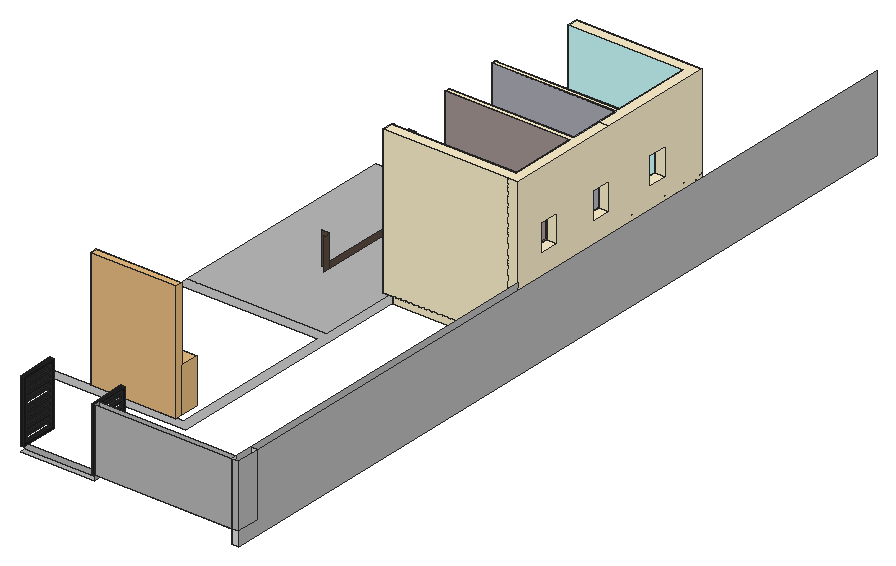
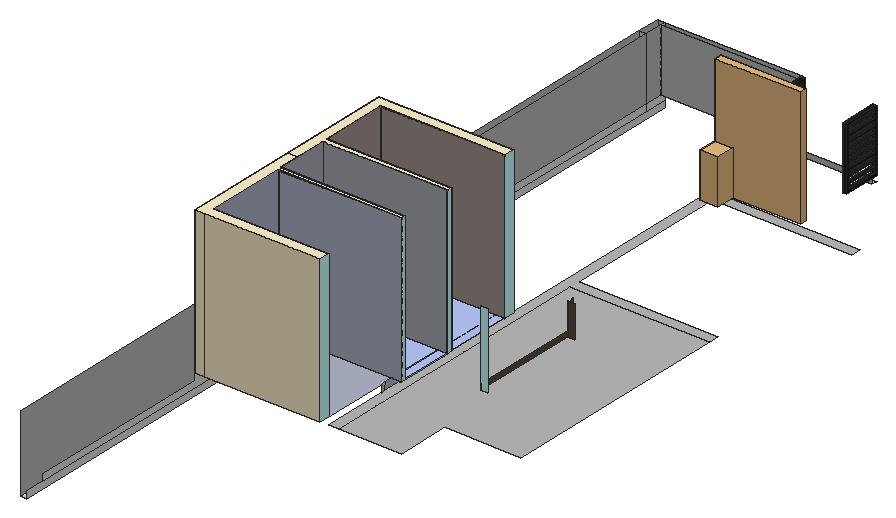
# SketchUp Ruby script. Lengths in inches.
U = 1.inch
M = Sketchup.active_model
def pt(a) = Geom::Point3d.new(a.map { |v| v * U })
def face(e, loops, mat)
  f = e.add_face(loops[0].map { |a| pt(a) })
  loops[1..].each { |l| e.add_face(l.map { |a| pt(a) }).erase! }
  f.material = f.back_material = mat if mat
  f
end
# faces: each face lists its corners as indices into pts; further lists are holes
def faces(e, pts, list, mat = nil) = list.each { |f| face(e, (f[0].is_a?(Array) ? f : [f]).map { |l| l.map { |i| pts[i] } }, mat) }
# xy, xz, yz: faces in a plane at the given z, y or x. An outline is a flat list of corners, or four numbers for a rectangle; further outlines are holes
def ring(l) = l.size == 4 ? [[l[0], l[1]], [l[2], l[1]], [l[2], l[3]], [l[0], l[3]]] : l.each_slice(2).to_a
def flat(e, list, mat, &to3) = list.each { |f| face(e, (f[0].is_a?(Array) ? f : [f]).map { |l| ring(l).map { |u, v| to3.(u, v) } }, mat) }
def xy(e, z, list, mat = nil) = flat(e, list, mat) { |x, y| [x, y, z] }
def xz(e, y, list, mat = nil) = flat(e, list, mat) { |x, z| [x, y, z] }
def yz(e, x, list, mat = nil) = flat(e, list, mat) { |y, z| [x, y, z] }
def lines(e, pts, list) = list.each { |a, b| e.add_line(pt(pts[a]), pt(pts[b])) }
# prism: a flat outline (further loops are holes) pulled along v
def prism(e, loops, v, mat = nil)
  f = face(e, loops, mat); d = Geom::Vector3d.new(v.map { |x| x * U })
  f.pushpull(f.normal.samedirection?(d) ? d.length : -d.length)
end
def box(e, o, s, mat = nil) = prism(e, [[o, [o[0] + s[0], o[1], o[2]], [o[0] + s[0], o[1] + s[1], o[2]], [o[0], o[1] + s[1], o[2]]]], [0, 0, s[2]], mat)
def at(x, y, z, deg = 0) = Geom::Transformation.translation(pt([x, y, z])) * Geom::Transformation.rotation(ORIGIN, Z_AXIS, deg.degrees)
def axes(o, x, y, z) = Geom::Transformation.new([*x, 0, *y, 0, *z, 0, *pt(o).to_a, 1])
def part(name) = M.definitions.add(name)
# library, detail: a bought-in or finely detailed component or shape, given as its bounding box
def library(name, o, s) = part(name).tap { |d| box(d.entities, o, s) }
def detail(e, o, s) = box(e.add_group.entities, o, s)
def put(e, d, t, mat = nil) = e.add_instance(d, t).tap { |i| i.material = mat if mat }
def group(e, t, mat = nil) = e.add_group.tap { |g| g.transformation = t; g.material = mat if mat }.entities
root = M.entities
M.materials.add("Brick_Stack_Bond_2K2").color = [186, 186, 186]
M.materials.add("D01_Frost_White").color = [255, 242, 206]
M.materials.add("Glass_Basic_01").color = [161, 173, 186]
M.materials["Glass_Basic_01"].alpha = 0.81
M.materials.add("Grid_20x20_1K").color = [185, 200, 252]
M.materials.add("H01_Misty_Ice1").color = [204, 255, 255]
M.materials.add("M01_Silver_Fog").color = [224, 224, 224]
M.materials.add("M02_Ash_Whisper").color = [196, 196, 196]
M.materials.add("M03_Pewter_Shine").color = [168, 168, 168]
M.materials.add("M08_Obsidian_Black").color = [30, 30, 30]
M.materials.add("Marble_03_1K").color = [175, 182, 201]
M.materials.add("Marble_06_1K").color = [165, 150, 147]
M.materials.add("Marble_20_1K").color = [172, 173, 182]
M.materials.add("Wood_Floor_12_1K").color = [92, 75, 65]
c1 = library("Group\#147",[0,0,0],[73.5,6.3125,102])
c2 = part("Group\#301")
xy(c2.entities,0,[[0,-3,32.08,0]],"M08_Obsidian_Black")
xy(c2.entities,2,[[2,-3,30.08,0]],"M08_Obsidian_Black")
xy(c2.entities,6.61,[[2,-3,30.08,0]],"M08_Obsidian_Black")
xy(c2.entities,7.61,[[2,-3,30.08,0]],"M08_Obsidian_Black")
xy(c2.entities,11.84,[[2,-3,30.08,0]],"M08_Obsidian_Black")
xy(c2.entities,12.84,[[2,-3,30.08,0]],"M08_Obsidian_Black")
xy(c2.entities,17.08,[[2,-3,30.08,0]],"M08_Obsidian_Black")
xy(c2.entities,18.08,[[2,-3,30.08,0]],"M08_Obsidian_Black")
xy(c2.entities,22.3125,[[2,-3,30.08,0]],"M08_Obsidian_Black")
xy(c2.entities,23.3125,[[2,-3,30.08,0]],"M08_Obsidian_Black")
xy(c2.entities,27.55,[[2,-3,30.08,0]],"M08_Obsidian_Black")
xy(c2.entities,28.55,[[2,-3,30.08,0]],"M08_Obsidian_Black")
xy(c2.entities,32.78,[[2,-3,30.08,0]],"M08_Obsidian_Black")
xy(c2.entities,33.78,[[2,-3,30.08,0]],"M08_Obsidian_Black")
xy(c2.entities,38.01,[[2,-3,30.08,0]],"M08_Obsidian_Black")
xy(c2.entities,39.01,[[2,-3,30.08,0]],"M08_Obsidian_Black")
xy(c2.entities,43.25,[[2,-3,30.08,0]],"M08_Obsidian_Black")
xy(c2.entities,44.25,[[2,-3,30.08,0]],"M08_Obsidian_Black")
xy(c2.entities,48.48,[[2,-3,30.08,0]],"M08_Obsidian_Black")
xy(c2.entities,49.48,[[2,-3,30.08,0]],"M08_Obsidian_Black")
xy(c2.entities,52,[[2,-3,30.08,0]],"M08_Obsidian_Black")
xy(c2.entities,54,[[0,-3,32.08,0]],"M08_Obsidian_Black")
xz(c2.entities,-3,[[[0,0,32.08,54],[2,2,30.08,52]],[2,6.61,30.08,7.61],[2,11.84,30.08,12.84],[2,17.08,30.08,18.08],[2,22.3125,30.08,23.3125],
  [2,27.55,30.08,28.55],[2,32.78,30.08,33.78],[2,38.01,30.08,39.01],[2,43.25,30.08,44.25],[2,48.48,30.08,49.48]],"M08_Obsidian_Black")
xz(c2.entities,0,[[[0,0,0,54,32.08,54,32.08,49.48,30.08,49.48,30.08,52,2,52,2,49.48,32.08,49.48,32.08,0],[2,2,30.08,6.61],[2,44.25,30.08,48.48],[2,33.78,30.08,38.01],[2,28.55,30.08,32.78],[2,23.3125,30.08,27.55],[2,18.08,30.08,22.3125],[2,12.84,30.08,17.08],[2,7.61,30.08,11.84],[2,39.01,30.08,43.25]]],"M08_Obsidian_Black")
yz(c2.entities,0,[[-3,0,0,54]],"M08_Obsidian_Black")
yz(c2.entities,2,[[-3,2,0,6.61],[-3,7.61,0,11.84],[-3,12.84,0,17.08],[-3,18.08,0,22.3125],[-3,23.3125,0,27.55],
  [-3,28.55,0,32.78],[-3,33.78,0,38.01],[-3,39.01,0,43.25],[-3,44.25,0,48.48],[-3,49.48,0,52]],"M08_Obsidian_Black")
yz(c2.entities,30.08,[[-3,2,0,6.61],[-3,7.61,0,11.84],[-3,12.84,0,17.08],[-3,18.08,0,22.3125],[-3,23.3125,0,27.55],
  [-3,28.55,0,32.78],[-3,33.78,0,38.01],[-3,39.01,0,43.25],[-3,44.25,0,48.48],[-3,49.48,0,52]],"M08_Obsidian_Black")
yz(c2.entities,32.08,[[-3,0,0,52],[-3,52,0,54]],"M08_Obsidian_Black")
c3 = library("Group\#155",[0,0,0],[19.75,19.75,54.55])
xy(root,0,[[2047.75,129.625,2053.75,815.6875]],"M01_Silver_Fog")
xy(root,7.5,[[1865.79,129.625,1929.96,134.375]],"Brick_Stack_Bond_2K2")
xy(root,12,[[1810.75,215.6875,1939.75,215.6875,1939.75,626.6875,1930.75,626.6875,1930.75,377.6875,1810.75,377.6875,1810.75,368.6875,1930.75,368.6875,1930.75,224.6875,1810.75,224.6875],[1810.75,377.6875,1930.75,377.6875,1930.75,626.6875,1876.75,626.6875,1876.75,580.6875,1810.75,580.6875]],"Brick_Stack_Bond_2K2")
xy(root,12,[[1929.96,129.625,2047.75,134.375],[2047.75,129.625,2053.75,149.6875]],"M01_Silver_Fog")
xz(root,129.625,[[1929.96,12,2047.75,66],[2047.75,12,2053.75,66]],"Brick_Stack_Bond_2K2")
xz(root,129.625,[[2047.75,0,2053.75,12]],"M01_Silver_Fog")
xz(root,134.375,[[1865.79,7.5,1929.96,12],[1929.96,12,2047.75,66]],"Brick_Stack_Bond_2K2")
xz(root,149.6875,[[2047.75,12,2053.75,66]],"M01_Silver_Fog")
xz(root,437.6875,[[1939.75,12,2038.75,18],[2038.75,12,2047.75,18]],"D01_Frost_White")
xz(root,440.3125,[[1876.75,18,1882.75,45.8125]],"Wood_Floor_12_1K")
xz(root,533.5,[[1876.75,18,1882.75,82.875]],"H01_Misty_Ice1")
yz(root,1882.75,[[435.3125,18,440.3125,18,440.3125,45.8125,437.79,43.29,435.3125,45.77],[440.3125,18,533.5,23]],"Wood_Floor_12_1K")
yz(root,1929.96,[[129.625,7.5,134.375,12],[129.625,12,134.375,66]],"M03_Pewter_Shine")
yz(root,1939.75,[[437.6875,12,446.6875,18],[504.6875,12,508.6875,18],[565.6875,12,569.6875,18]],"Brick_Stack_Bond_2K2")
yz(root,1939.75,[[446.6875,12,504.6875,18],[508.6875,12,565.6875,18]],"Marble_03_1K")
yz(root,2047.75,[[134.375,12,149.6875,66],[149.6875,12,437.6875,66]],"Brick_Stack_Bond_2K2")
yz(root,2047.75,[[129.625,0,815.6875,6],[129.625,6,149.6875,12],[149.6875,6,149.6875,12,437.6875,12,437.6875,66,635.6875,66,635.6875,12,798.625,12,798.625,6],[129.625,12,134.375,66]],"M01_Silver_Fog")
yz(root,2053.75,[[129.625,0,815.6875,0,815.6875,66,149.6875,66,149.6875,12,129.625,12],[129.625,12,149.6875,66]],"Brick_Stack_Bond_2K2")
put(root,c1,at(1857.25,215.6875,18),"Glass_Basic_01")
g1 = group(root,at(1865.79,129.625,12))
put(g1,c2,at(61.17,0,0,90))
put(g1,c2,at(0,0,0,90))
put(root,c3,axes([1915.35,221.6875,18],[0.78,0,0],[0,0.847,0],[0,0,0.704]))
g2 = group(root,at(1939.75,557.8125,18),"M02_Ash_Whisper")
prism(g2,[[[97.07,0.01,0],[-8.0625,0,0],[-8.0625,0.375,0],[97.07,0.39,0]]],[0,0,126],"Marble_03_1K")
g3 = group(root,at(1939.75,446.6875,18),"Marble_06_1K")
box(g3,[-8.0625,0,0],[106.6875,0.25,126])
g4 = group(root,at(1939.75,504.6875,18),"M02_Ash_Whisper")
box(g4,[-8.0625,-0.3125,0],[107.0625,0.3125,126],"Marble_06_1K")
g5 = group(root,at(1939.75,508.6875,18),"M02_Ash_Whisper")
box(g5,[-8.0625,0,0],[107.0625,0.15,126],"Marble_20_1K")
g6 = group(root,at(1939.75,554.4375,18),"M02_Ash_Whisper")
box(g6,[-8.0625,-0.16,0],[107.0625,0.16,126],"Marble_20_1K")
g7 = group(root,at(1939.75,437.6875,18),"Brick_Stack_Bond_2K2")
xy(g7,0,[[-8.0625,71,99,116.75]],"Grid_20x20_1K")
xy(g7,0,[[-8.0625,0,-8.0625,9,99,9,99,67,-8.0625,67,-8.0625,71,99,71,99,116.75,-8.0625,116.75,-8.0625,120.125,98.3125,120.125,98.3125,189,0,189,0,198,108,198,108,0]],"H01_Misty_Ice1")
xy(g7,0,[[0,120.125,98.3125,189]],"Marble_03_1K")
xy(g7,0.25,[[-8.0625,9,99,67],[-8.0625,71,99,116.75]],"Grid_20x20_1K")
xy(g7,60,[[99,24,108,42],[99,80.1875,108,98.1875],[98.3125,140.8125,108,158.8125]],"D01_Frost_White")
xy(g7,84,[[99,24,108,42],[99,80.1875,108,98.1875],[98.3125,140.8125,108,158.8125]],"D01_Frost_White")
xy(g7,126,[[-8.0625,0,108,0,108,98.1875,99,98.1875,99,71,-8.0625,71,-8.0625,67,99,67,99,9,-8.0625,9],[99,98.1875,108,98.1875,108,198,0,198,0,189,98.3125,189,98.3125,120.125,-8.0625,120.125,-8.0625,116.75,99,116.75]],"D01_Frost_White")
xz(g7,0,[[-8.0625,0,99,126],[99,0,108,126]],"D01_Frost_White")
xz(g7,9,[[-8.0625,0,99,0.25]],"Grid_20x20_1K")
xz(g7,9,[[-8.0625,0.25,99,126]],"H01_Misty_Ice1")
xz(g7,24,[[99,60,108,84]],"D01_Frost_White")
xz(g7,42,[[99,60,108,84]],"D01_Frost_White")
xz(g7,67,[[-8.0625,0,99,0.25]],"Grid_20x20_1K")
xz(g7,67,[[-8.0625,0.25,99,126]],"H01_Misty_Ice1")
xz(g7,71,[[-8.0625,0,99,0.25]],"Grid_20x20_1K")
xz(g7,71,[[-8.0625,0.25,99,126]],"H01_Misty_Ice1")
xz(g7,80.1875,[[99,60,108,84]],"D01_Frost_White")
xz(g7,98.1875,[[99,60,108,84]],"D01_Frost_White")
xz(g7,116.75,[[-8.0625,0,99,0.25]],"Grid_20x20_1K")
xz(g7,116.75,[[-8.0625,0.25,99,126]],"H01_Misty_Ice1")
xz(g7,120.125,[[-8.0625,0,98.3125,126]],"H01_Misty_Ice1")
xz(g7,140.8125,[[98.3125,60,108,84]],"D01_Frost_White")
xz(g7,158.8125,[[98.3125,60,108,84]],"D01_Frost_White")
xz(g7,189,[[0,0,98.3125,126]],"H01_Misty_Ice1")
xz(g7,198,[[0,0,99,126],[99,0,108,126]],"D01_Frost_White")
yz(g7,-8.0625,[[9,0,67,0.25],[71,0,116.75,0.25]],"Grid_20x20_1K")
yz(g7,-8.0625,[[0,0,9,126],[67,0,71,126],[116.75,0,120.125,126]],"H01_Misty_Ice1")
yz(g7,0,[[189,0,198,126]],"H01_Misty_Ice1")
yz(g7,98.3125,[[[120.125,0,189,126],[140.8125,60,158.8125,84]]],"Marble_03_1K")
yz(g7,99,[[9,0,67,0.25],[71,0,116.75,0.25]],"Grid_20x20_1K")
yz(g7,99,[[[9,0.25,67,126],[24,60,42,84]],[[71,0.25,116.75,126],[80.1875,60,98.1875,84]]],"H01_Misty_Ice1")
yz(g7,108,[[[0,0,198,126],[140.8125,60,158.8125,84],[80.1875,60,98.1875,84],[24,60,42,84]]],"D01_Frost_White")
p = [[99,80.1875,126],[98.79,80.1875,126]]
lines(g7,p,[[0,1]])
g8 = group(root,at(2038.75,446.6875,18),"M02_Ash_Whisper")
prism(g8,[[[-0.375,0,126],[-0.375,57.6875,126],[-0.375,57.6875,0],[-0.375,0,0]],[[-0.375,33,60],[-0.375,33,84],[-0.375,15,84],[-0.375,15,60]]],[0.375,0,0],"Marble_06_1K")
g9 = group(root,at(2038.75,508.84,18),"M02_Ash_Whisper")
prism(g9,[[[0,45.4375,0],[0,45.4375,126],[0,0,126],[0,0,0]],[[0,27.04,60],[0,9.04,60],[0,9.04,84],[0,27.04,84]]],[-0.21,0,0],"Marble_20_1K")
